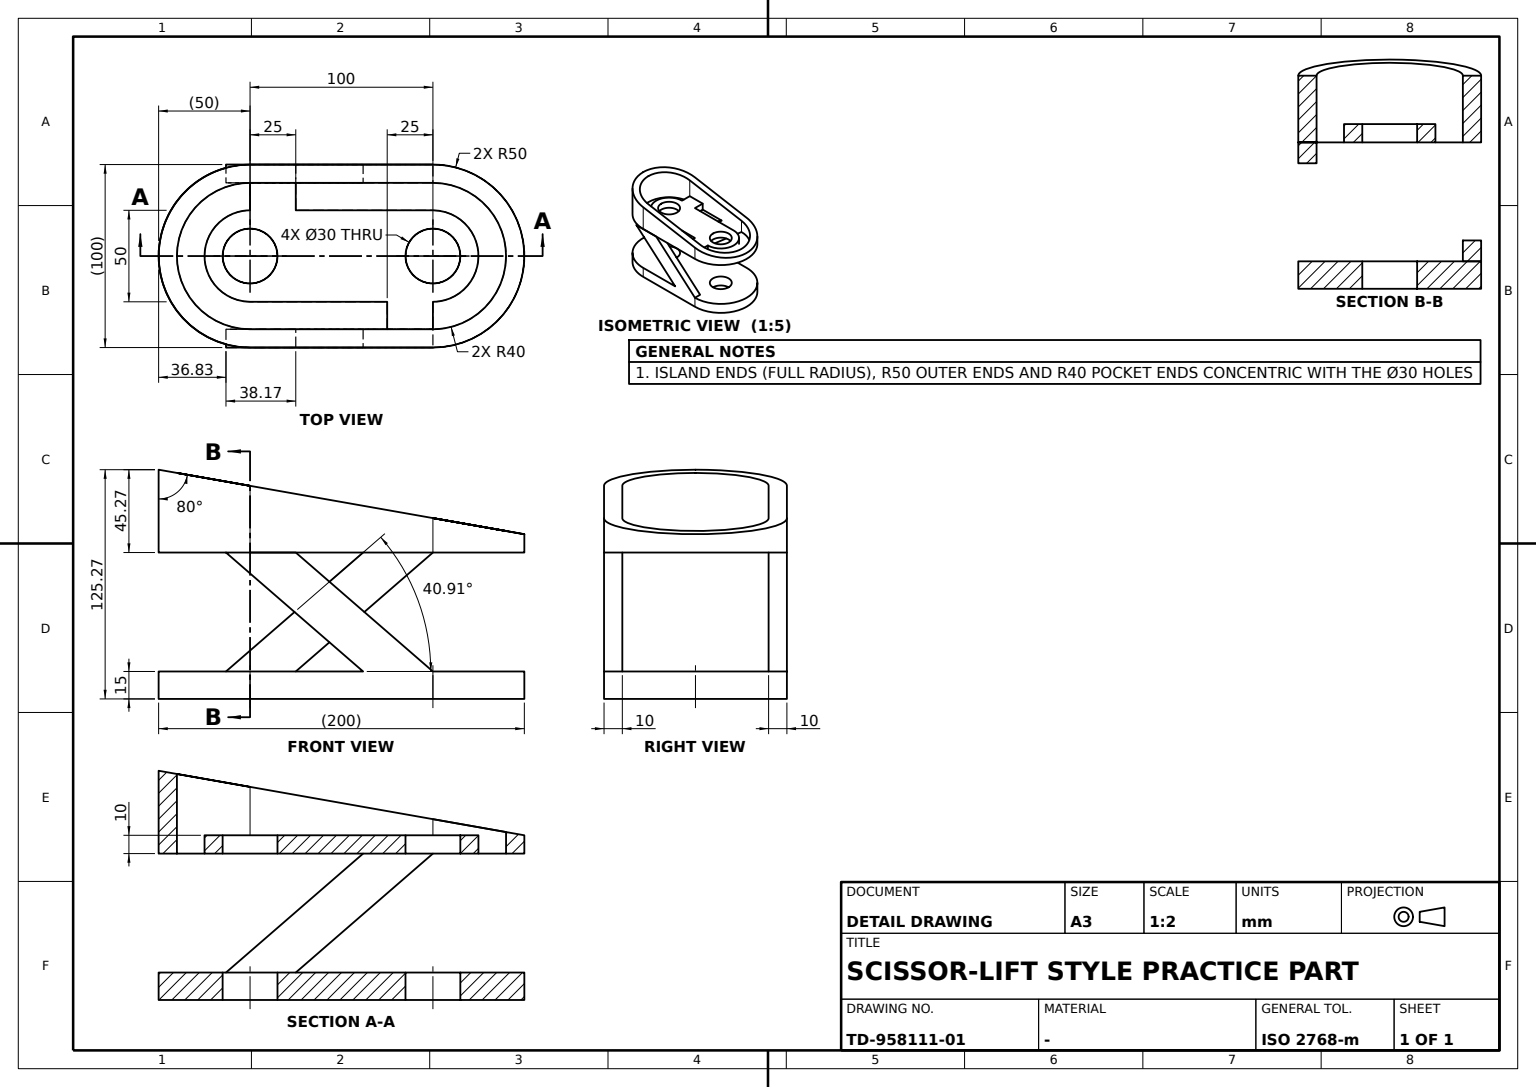
ISO-10303-21;
HEADER;
FILE_DESCRIPTION((''),'2;1');
FILE_NAME('','',(''),(''),'','','');
FILE_SCHEMA(('AUTOMOTIVE_DESIGN'));
ENDSEC;
DATA;
#1=APPLICATION_CONTEXT('');
#2=PRODUCT_CONTEXT('',#1,'mechanical');
#3=PRODUCT('','','',(#2));
#4=PRODUCT_DEFINITION_FORMATION('','',#3);
#5=PRODUCT_DEFINITION_CONTEXT('',#1,'design');
#6=PRODUCT_DEFINITION('','',#4,#5);
#7=PRODUCT_DEFINITION_SHAPE('','',#6);
#8=(LENGTH_UNIT()NAMED_UNIT(*)SI_UNIT(.MILLI.,.METRE.));
#9=(NAMED_UNIT(*)PLANE_ANGLE_UNIT()SI_UNIT($,.RADIAN.));
#10=(NAMED_UNIT(*)SI_UNIT($,.STERADIAN.)SOLID_ANGLE_UNIT());
#11=UNCERTAINTY_MEASURE_WITH_UNIT(LENGTH_MEASURE(0.005),#8,'distance_accuracy_value','');
#12=(GEOMETRIC_REPRESENTATION_CONTEXT(3)GLOBAL_UNCERTAINTY_ASSIGNED_CONTEXT((#11))GLOBAL_UNIT_ASSIGNED_CONTEXT((#8,#9,#10))REPRESENTATION_CONTEXT('',''));
#13=CARTESIAN_POINT('',(50.,-50.,0.));
#14=VERTEX_POINT('',#13);
#15=CARTESIAN_POINT('',(100.,0.,0.));
#16=VERTEX_POINT('',#15);
#17=CARTESIAN_POINT('',(50.,0.,0.));
#18=DIRECTION('',(0.,0.,1.));
#19=DIRECTION('',(1.,0.,0.));
#20=AXIS2_PLACEMENT_3D('',#17,#18,#19);
#21=CIRCLE('',#20,50.);
#22=EDGE_CURVE('',#14,#16,#21,.T.);
#23=ORIENTED_EDGE('',*,*,#22,.F.);
#24=CARTESIAN_POINT('',(50.,-50.,-15.));
#25=VERTEX_POINT('',#24);
#26=VECTOR('',#18,1000.);
#27=LINE('',#24,#26);
#28=EDGE_CURVE('',#25,#14,#27,.T.);
#29=ORIENTED_EDGE('',*,*,#28,.F.);
#30=CARTESIAN_POINT('',(100.,0.,-15.));
#31=VERTEX_POINT('',#30);
#32=CARTESIAN_POINT('',(50.,0.,-15.));
#33=AXIS2_PLACEMENT_3D('',#32,#18,#19);
#34=CIRCLE('',#33,50.);
#35=EDGE_CURVE('',#25,#31,#34,.T.);
#36=ORIENTED_EDGE('',*,*,#35,.T.);
#37=LINE('',#30,#26);
#38=EDGE_CURVE('',#31,#16,#37,.T.);
#39=ORIENTED_EDGE('',*,*,#38,.T.);
#40=EDGE_LOOP('',(#23,#29,#36,#39));
#41=FACE_BOUND('',#40,.T.);
#42=CYLINDRICAL_SURFACE('',#33,50.);
#43=ADVANCED_FACE('',(#41),#42,.T.);
#44=CARTESIAN_POINT('',(-65.,0.,0.));
#45=VERTEX_POINT('',#44);
#46=CARTESIAN_POINT('',(-35.,0.,0.));
#47=VERTEX_POINT('',#46);
#48=CARTESIAN_POINT('',(-50.,0.,0.));
#49=AXIS2_PLACEMENT_3D('',#48,#18,#19);
#50=CIRCLE('',#49,15.);
#51=EDGE_CURVE('',#45,#47,#50,.T.);
#52=ORIENTED_EDGE('',*,*,#51,.T.);
#53=CARTESIAN_POINT('',(-35.,0.,-15.));
#54=VERTEX_POINT('',#53);
#55=LINE('',#53,#26);
#56=EDGE_CURVE('',#54,#47,#55,.T.);
#57=ORIENTED_EDGE('',*,*,#56,.F.);
#58=CARTESIAN_POINT('',(-65.,0.,-15.));
#59=VERTEX_POINT('',#58);
#60=CARTESIAN_POINT('',(-50.,0.,-15.));
#61=AXIS2_PLACEMENT_3D('',#60,#18,#19);
#62=CIRCLE('',#61,15.);
#63=EDGE_CURVE('',#59,#54,#62,.T.);
#64=ORIENTED_EDGE('',*,*,#63,.F.);
#65=LINE('',#58,#26);
#66=EDGE_CURVE('',#45,#59,#65,.F.);
#67=ORIENTED_EDGE('',*,*,#66,.F.);
#68=EDGE_LOOP('',(#52,#57,#64,#67));
#69=FACE_BOUND('',#68,.T.);
#70=CYLINDRICAL_SURFACE('',#61,15.);
#71=ADVANCED_FACE('',(#69),#70,.F.);
#72=CARTESIAN_POINT('',(-63.171987,-50.,65.));
#73=VERTEX_POINT('',#72);
#74=CARTESIAN_POINT('',(11.828013,-50.,0.));
#75=VERTEX_POINT('',#74);
#76=DIRECTION('',(0.755689083,0.,-0.654930538));
#77=VECTOR('',#76,1000.);
#78=LINE('',#72,#77);
#79=EDGE_CURVE('',#73,#75,#78,.T.);
#80=ORIENTED_EDGE('',*,*,#79,.F.);
#81=CARTESIAN_POINT('',(-63.171987,-40.,65.));
#82=VERTEX_POINT('',#81);
#83=DIRECTION('',(0.,-1.,0.));
#84=VECTOR('',#83,1000.);
#85=LINE('',#81,#84);
#86=EDGE_CURVE('',#82,#73,#85,.T.);
#87=ORIENTED_EDGE('',*,*,#86,.F.);
#88=CARTESIAN_POINT('',(11.828013,-40.,0.));
#89=VERTEX_POINT('',#88);
#90=LINE('',#81,#77);
#91=EDGE_CURVE('',#82,#89,#90,.T.);
#92=ORIENTED_EDGE('',*,*,#91,.T.);
#93=LINE('',#88,#84);
#94=EDGE_CURVE('',#89,#75,#93,.T.);
#95=ORIENTED_EDGE('',*,*,#94,.T.);
#96=EDGE_LOOP('',(#80,#87,#92,#95));
#97=FACE_BOUND('',#96,.T.);
#98=DIRECTION('',(-0.654930538,0.,-0.755689083));
#99=DIRECTION('',(-0.755689083,0.,0.654930538));
#100=AXIS2_PLACEMENT_3D('',#81,#98,#99);
#101=PLANE('',#100);
#102=ADVANCED_FACE('',(#97),#101,.T.);
#103=CARTESIAN_POINT('',(50.,50.,-15.));
#104=VERTEX_POINT('',#103);
#105=CARTESIAN_POINT('',(-50.,50.,-15.));
#106=VERTEX_POINT('',#105);
#107=DIRECTION('',(-1.,0.,0.));
#108=VECTOR('',#107,1000.);
#109=LINE('',#103,#108);
#110=EDGE_CURVE('',#104,#106,#109,.T.);
#111=ORIENTED_EDGE('',*,*,#110,.T.);
#112=CARTESIAN_POINT('',(-50.,50.,0.));
#113=VERTEX_POINT('',#112);
#114=LINE('',#105,#26);
#115=EDGE_CURVE('',#106,#113,#114,.T.);
#116=ORIENTED_EDGE('',*,*,#115,.T.);
#117=CARTESIAN_POINT('',(50.,50.,0.));
#118=VERTEX_POINT('',#117);
#119=LINE('',#117,#108);
#120=EDGE_CURVE('',#118,#113,#119,.T.);
#121=ORIENTED_EDGE('',*,*,#120,.F.);
#122=LINE('',#103,#26);
#123=EDGE_CURVE('',#104,#118,#122,.T.);
#124=ORIENTED_EDGE('',*,*,#123,.F.);
#125=EDGE_LOOP('',(#111,#116,#121,#124));
#126=FACE_BOUND('',#125,.T.);
#127=DIRECTION('',(0.,1.,0.));
#128=AXIS2_PLACEMENT_3D('',#103,#127,#18);
#129=PLANE('',#128);
#130=ADVANCED_FACE('',(#126),#129,.T.);
#131=CARTESIAN_POINT('',(-50.,-50.,-15.));
#132=VERTEX_POINT('',#131);
#133=CIRCLE('',#61,50.);
#134=EDGE_CURVE('',#106,#132,#133,.T.);
#135=ORIENTED_EDGE('',*,*,#134,.T.);
#136=CARTESIAN_POINT('',(-50.,-50.,0.));
#137=VERTEX_POINT('',#136);
#138=LINE('',#131,#26);
#139=EDGE_CURVE('',#132,#137,#138,.T.);
#140=ORIENTED_EDGE('',*,*,#139,.T.);
#141=CIRCLE('',#49,50.);
#142=EDGE_CURVE('',#113,#137,#141,.T.);
#143=ORIENTED_EDGE('',*,*,#142,.F.);
#144=ORIENTED_EDGE('',*,*,#115,.F.);
#145=EDGE_LOOP('',(#135,#140,#143,#144));
#146=FACE_BOUND('',#145,.T.);
#147=CYLINDRICAL_SURFACE('',#61,50.);
#148=ADVANCED_FACE('',(#146),#147,.T.);
#149=CARTESIAN_POINT('',(65.,0.,0.));
#150=VERTEX_POINT('',#149);
#151=CARTESIAN_POINT('',(35.,0.,0.));
#152=VERTEX_POINT('',#151);
#153=CIRCLE('',#20,15.);
#154=EDGE_CURVE('',#150,#152,#153,.T.);
#155=ORIENTED_EDGE('',*,*,#154,.T.);
#156=CARTESIAN_POINT('',(35.,0.,-15.));
#157=VERTEX_POINT('',#156);
#158=LINE('',#156,#26);
#159=EDGE_CURVE('',#152,#157,#158,.F.);
#160=ORIENTED_EDGE('',*,*,#159,.T.);
#161=CARTESIAN_POINT('',(65.,0.,-15.));
#162=VERTEX_POINT('',#161);
#163=CIRCLE('',#33,15.);
#164=EDGE_CURVE('',#162,#157,#163,.T.);
#165=ORIENTED_EDGE('',*,*,#164,.F.);
#166=LINE('',#161,#26);
#167=EDGE_CURVE('',#162,#150,#166,.T.);
#168=ORIENTED_EDGE('',*,*,#167,.T.);
#169=EDGE_LOOP('',(#155,#160,#165,#168));
#170=FACE_BOUND('',#169,.T.);
#171=CYLINDRICAL_SURFACE('',#33,15.);
#172=ADVANCED_FACE('',(#170),#171,.F.);
#173=CARTESIAN_POINT('',(-25.,-50.,65.));
#174=VERTEX_POINT('',#173);
#175=LINE('',#173,#108);
#176=EDGE_CURVE('',#174,#73,#175,.T.);
#177=ORIENTED_EDGE('',*,*,#176,.F.);
#178=CARTESIAN_POINT('',(-25.,-40.,65.));
#179=VERTEX_POINT('',#178);
#180=LINE('',#178,#84);
#181=EDGE_CURVE('',#179,#174,#180,.T.);
#182=ORIENTED_EDGE('',*,*,#181,.F.);
#183=LINE('',#178,#108);
#184=EDGE_CURVE('',#179,#82,#183,.T.);
#185=ORIENTED_EDGE('',*,*,#184,.T.);
#186=ORIENTED_EDGE('',*,*,#86,.T.);
#187=EDGE_LOOP('',(#177,#182,#185,#186));
#188=FACE_BOUND('',#187,.T.);
#189=AXIS2_PLACEMENT_3D('',#178,#18,#19);
#190=PLANE('',#189);
#191=ADVANCED_FACE('',(#188),#190,.T.);
#192=ORIENTED_EDGE('',*,*,#181,.T.);
#193=VECTOR('',#99,1000.);
#194=LINE('',#13,#193);
#195=EDGE_CURVE('',#14,#174,#194,.T.);
#196=ORIENTED_EDGE('',*,*,#195,.F.);
#197=CARTESIAN_POINT('',(50.,-40.,0.));
#198=VERTEX_POINT('',#197);
#199=LINE('',#197,#84);
#200=EDGE_CURVE('',#198,#14,#199,.T.);
#201=ORIENTED_EDGE('',*,*,#200,.F.);
#202=LINE('',#197,#193);
#203=EDGE_CURVE('',#198,#179,#202,.T.);
#204=ORIENTED_EDGE('',*,*,#203,.T.);
#205=EDGE_LOOP('',(#192,#196,#201,#204));
#206=FACE_BOUND('',#205,.T.);
#207=DIRECTION('',(0.654930538,0.,0.755689083));
#208=AXIS2_PLACEMENT_3D('',#197,#207,#76);
#209=PLANE('',#208);
#210=ADVANCED_FACE('',(#206),#209,.T.);
#211=EDGE_CURVE('',#54,#59,#62,.T.);
#212=ORIENTED_EDGE('',*,*,#211,.T.);
#213=ORIENTED_EDGE('',*,*,#63,.T.);
#214=EDGE_LOOP('',(#212,#213));
#215=FACE_BOUND('',#214,.T.);
#216=ORIENTED_EDGE('',*,*,#35,.F.);
#217=VECTOR('',#19,1000.);
#218=LINE('',#131,#217);
#219=EDGE_CURVE('',#132,#25,#218,.T.);
#220=ORIENTED_EDGE('',*,*,#219,.F.);
#221=ORIENTED_EDGE('',*,*,#134,.F.);
#222=ORIENTED_EDGE('',*,*,#110,.F.);
#223=EDGE_CURVE('',#31,#104,#34,.T.);
#224=ORIENTED_EDGE('',*,*,#223,.F.);
#225=EDGE_LOOP('',(#216,#220,#221,#222,#224));
#226=FACE_BOUND('',#225,.T.);
#227=EDGE_CURVE('',#157,#162,#163,.T.);
#228=ORIENTED_EDGE('',*,*,#227,.T.);
#229=ORIENTED_EDGE('',*,*,#164,.T.);
#230=EDGE_LOOP('',(#228,#229));
#231=FACE_BOUND('',#230,.T.);
#232=PLANE('',#61);
#233=ADVANCED_FACE('',(#215,#226,#231),#232,.F.);
#234=ORIENTED_EDGE('',*,*,#120,.T.);
#235=ORIENTED_EDGE('',*,*,#142,.T.);
#236=LINE('',#136,#217);
#237=EDGE_CURVE('',#137,#75,#236,.T.);
#238=ORIENTED_EDGE('',*,*,#237,.T.);
#239=ORIENTED_EDGE('',*,*,#94,.F.);
#240=LINE('',#88,#217);
#241=EDGE_CURVE('',#89,#198,#240,.T.);
#242=ORIENTED_EDGE('',*,*,#241,.T.);
#243=ORIENTED_EDGE('',*,*,#200,.T.);
#244=ORIENTED_EDGE('',*,*,#22,.T.);
#245=EDGE_CURVE('',#16,#118,#21,.T.);
#246=ORIENTED_EDGE('',*,*,#245,.T.);
#247=EDGE_LOOP('',(#234,#235,#238,#239,#242,#243,#244,#246));
#248=FACE_BOUND('',#247,.T.);
#249=ORIENTED_EDGE('',*,*,#51,.F.);
#250=EDGE_CURVE('',#47,#45,#50,.T.);
#251=ORIENTED_EDGE('',*,*,#250,.F.);
#252=EDGE_LOOP('',(#249,#251));
#253=FACE_BOUND('',#252,.T.);
#254=ORIENTED_EDGE('',*,*,#154,.F.);
#255=EDGE_CURVE('',#152,#150,#153,.T.);
#256=ORIENTED_EDGE('',*,*,#255,.F.);
#257=EDGE_LOOP('',(#254,#256));
#258=FACE_BOUND('',#257,.T.);
#259=PLANE('',#49);
#260=ADVANCED_FACE('',(#248,#253,#258),#259,.T.);
#261=ORIENTED_EDGE('',*,*,#123,.T.);
#262=ORIENTED_EDGE('',*,*,#245,.F.);
#263=ORIENTED_EDGE('',*,*,#38,.F.);
#264=ORIENTED_EDGE('',*,*,#223,.T.);
#265=EDGE_LOOP('',(#261,#262,#263,#264));
#266=FACE_BOUND('',#265,.T.);
#267=ADVANCED_FACE('',(#266),#42,.T.);
#268=ORIENTED_EDGE('',*,*,#167,.F.);
#269=ORIENTED_EDGE('',*,*,#227,.F.);
#270=ORIENTED_EDGE('',*,*,#159,.F.);
#271=ORIENTED_EDGE('',*,*,#255,.T.);
#272=EDGE_LOOP('',(#268,#269,#270,#271));
#273=FACE_BOUND('',#272,.T.);
#274=ADVANCED_FACE('',(#273),#171,.F.);
#275=ORIENTED_EDGE('',*,*,#56,.T.);
#276=ORIENTED_EDGE('',*,*,#250,.T.);
#277=ORIENTED_EDGE('',*,*,#66,.T.);
#278=ORIENTED_EDGE('',*,*,#211,.F.);
#279=EDGE_LOOP('',(#275,#276,#277,#278));
#280=FACE_BOUND('',#279,.T.);
#281=ADVANCED_FACE('',(#280),#70,.F.);
#282=ORIENTED_EDGE('',*,*,#28,.T.);
#283=ORIENTED_EDGE('',*,*,#195,.T.);
#284=ORIENTED_EDGE('',*,*,#176,.T.);
#285=ORIENTED_EDGE('',*,*,#79,.T.);
#286=ORIENTED_EDGE('',*,*,#237,.F.);
#287=ORIENTED_EDGE('',*,*,#139,.F.);
#288=ORIENTED_EDGE('',*,*,#219,.T.);
#289=EDGE_LOOP('',(#282,#283,#284,#285,#286,#287,#288));
#290=FACE_BOUND('',#289,.T.);
#291=DIRECTION('',(0.,0.,-1.));
#292=AXIS2_PLACEMENT_3D('',#131,#83,#291);
#293=PLANE('',#292);
#294=ADVANCED_FACE('',(#290),#293,.T.);
#295=ORIENTED_EDGE('',*,*,#241,.F.);
#296=ORIENTED_EDGE('',*,*,#91,.F.);
#297=ORIENTED_EDGE('',*,*,#184,.F.);
#298=ORIENTED_EDGE('',*,*,#203,.F.);
#299=EDGE_LOOP('',(#295,#296,#297,#298));
#300=FACE_BOUND('',#299,.T.);
#301=CARTESIAN_POINT('',(0.,-40.,0.));
#302=AXIS2_PLACEMENT_3D('',#301,#83,#291);
#303=PLANE('',#302);
#304=ADVANCED_FACE('',(#300),#303,.F.);
#305=CLOSED_SHELL('',(#43,#71,#102,#130,#148,#172,#191,#210,#233,#260,#267,#274,#281,#294,#304));
#306=MANIFOLD_SOLID_BREP('',#305);
#307=CARTESIAN_POINT('',(35.,0.,75.));
#308=VERTEX_POINT('',#307);
#309=CARTESIAN_POINT('',(65.,0.,75.));
#310=VERTEX_POINT('',#309);
#311=CARTESIAN_POINT('',(50.,0.,75.));
#312=AXIS2_PLACEMENT_3D('',#311,#18,#19);
#313=CIRCLE('',#312,15.);
#314=EDGE_CURVE('',#308,#310,#313,.T.);
#315=ORIENTED_EDGE('',*,*,#314,.T.);
#316=CARTESIAN_POINT('',(65.,0.,65.));
#317=VERTEX_POINT('',#316);
#318=LINE('',#316,#26);
#319=EDGE_CURVE('',#310,#317,#318,.F.);
#320=ORIENTED_EDGE('',*,*,#319,.T.);
#321=CARTESIAN_POINT('',(35.,0.,65.));
#322=VERTEX_POINT('',#321);
#323=CARTESIAN_POINT('',(50.,0.,65.));
#324=AXIS2_PLACEMENT_3D('',#323,#18,#19);
#325=CIRCLE('',#324,15.);
#326=EDGE_CURVE('',#322,#317,#325,.T.);
#327=ORIENTED_EDGE('',*,*,#326,.F.);
#328=LINE('',#321,#26);
#329=EDGE_CURVE('',#322,#308,#328,.T.);
#330=ORIENTED_EDGE('',*,*,#329,.T.);
#331=EDGE_LOOP('',(#315,#320,#327,#330));
#332=FACE_BOUND('',#331,.T.);
#333=CYLINDRICAL_SURFACE('',#324,15.);
#334=ADVANCED_FACE('',(#332),#333,.F.);
#335=CARTESIAN_POINT('',(-63.171987,50.,0.));
#336=VERTEX_POINT('',#335);
#337=CARTESIAN_POINT('',(11.828013,50.,65.));
#338=VERTEX_POINT('',#337);
#339=DIRECTION('',(0.755689083,0.,0.654930538));
#340=VECTOR('',#339,1000.);
#341=LINE('',#335,#340);
#342=EDGE_CURVE('',#336,#338,#341,.T.);
#343=ORIENTED_EDGE('',*,*,#342,.F.);
#344=CARTESIAN_POINT('',(-63.171987,40.,0.));
#345=VERTEX_POINT('',#344);
#346=VECTOR('',#127,1000.);
#347=LINE('',#344,#346);
#348=EDGE_CURVE('',#345,#336,#347,.T.);
#349=ORIENTED_EDGE('',*,*,#348,.F.);
#350=CARTESIAN_POINT('',(11.828013,40.,65.));
#351=VERTEX_POINT('',#350);
#352=LINE('',#344,#340);
#353=EDGE_CURVE('',#345,#351,#352,.T.);
#354=ORIENTED_EDGE('',*,*,#353,.T.);
#355=LINE('',#350,#346);
#356=EDGE_CURVE('',#351,#338,#355,.T.);
#357=ORIENTED_EDGE('',*,*,#356,.T.);
#358=EDGE_LOOP('',(#343,#349,#354,#357));
#359=FACE_BOUND('',#358,.T.);
#360=DIRECTION('',(-0.654930538,0.,0.755689083));
#361=AXIS2_PLACEMENT_3D('',#344,#360,#339);
#362=PLANE('',#361);
#363=ADVANCED_FACE('',(#359),#362,.T.);
#364=CARTESIAN_POINT('',(50.,40.,65.));
#365=VERTEX_POINT('',#364);
#366=CARTESIAN_POINT('',(50.,40.,83.816349));
#367=VERTEX_POINT('',#366);
#368=CARTESIAN_POINT('',(50.,40.,165.));
#369=LINE('',#368,#26);
#370=EDGE_CURVE('',#365,#367,#369,.T.);
#371=ORIENTED_EDGE('',*,*,#370,.T.);
#372=CARTESIAN_POINT('',(-50.,40.,101.449047));
#373=VERTEX_POINT('',#372);
#374=CARTESIAN_POINT('',(100.,40.,75.));
#375=DIRECTION('',(0.984807753,0.,-0.173648178));
#376=VECTOR('',#375,1000.);
#377=LINE('',#374,#376);
#378=EDGE_CURVE('',#373,#367,#377,.T.);
#379=ORIENTED_EDGE('',*,*,#378,.F.);
#380=CARTESIAN_POINT('',(-50.,40.,75.));
#381=VERTEX_POINT('',#380);
#382=CARTESIAN_POINT('',(-50.,40.,165.));
#383=LINE('',#382,#26);
#384=EDGE_CURVE('',#381,#373,#383,.T.);
#385=ORIENTED_EDGE('',*,*,#384,.F.);
#386=CARTESIAN_POINT('',(-25.,40.,75.));
#387=VERTEX_POINT('',#386);
#388=LINE('',#380,#217);
#389=EDGE_CURVE('',#381,#387,#388,.T.);
#390=ORIENTED_EDGE('',*,*,#389,.T.);
#391=CARTESIAN_POINT('',(-25.,40.,65.));
#392=VERTEX_POINT('',#391);
#393=VECTOR('',#291,1000.);
#394=LINE('',#386,#393);
#395=EDGE_CURVE('',#387,#392,#394,.T.);
#396=ORIENTED_EDGE('',*,*,#395,.T.);
#397=CARTESIAN_POINT('',(-50.,40.,65.));
#398=LINE('',#397,#217);
#399=EDGE_CURVE('',#392,#351,#398,.T.);
#400=ORIENTED_EDGE('',*,*,#399,.T.);
#401=ORIENTED_EDGE('',*,*,#353,.F.);
#402=CARTESIAN_POINT('',(-25.,40.,0.));
#403=VERTEX_POINT('',#402);
#404=LINE('',#402,#108);
#405=EDGE_CURVE('',#403,#345,#404,.T.);
#406=ORIENTED_EDGE('',*,*,#405,.F.);
#407=DIRECTION('',(-0.755689083,0.,-0.654930538));
#408=VECTOR('',#407,1000.);
#409=LINE('',#364,#408);
#410=EDGE_CURVE('',#365,#403,#409,.T.);
#411=ORIENTED_EDGE('',*,*,#410,.F.);
#412=EDGE_LOOP('',(#371,#379,#385,#390,#396,#400,#401,#406,#411));
#413=FACE_BOUND('',#412,.T.);
#414=AXIS2_PLACEMENT_3D('',#382,#127,#107);
#415=PLANE('',#414);
#416=ADVANCED_FACE('',(#413),#415,.F.);
#417=ORIENTED_EDGE('',*,*,#326,.T.);
#418=EDGE_CURVE('',#317,#322,#325,.T.);
#419=ORIENTED_EDGE('',*,*,#418,.T.);
#420=EDGE_LOOP('',(#417,#419));
#421=FACE_BOUND('',#420,.T.);
#422=CARTESIAN_POINT('',(-50.,50.,65.));
#423=VERTEX_POINT('',#422);
#424=CARTESIAN_POINT('',(-100.,0.,65.));
#425=VERTEX_POINT('',#424);
#426=CARTESIAN_POINT('',(-50.,0.,65.));
#427=AXIS2_PLACEMENT_3D('',#426,#18,#107);
#428=CIRCLE('',#427,50.);
#429=EDGE_CURVE('',#423,#425,#428,.T.);
#430=ORIENTED_EDGE('',*,*,#429,.F.);
#431=CARTESIAN_POINT('',(-100.,50.,65.));
#432=LINE('',#431,#217);
#433=EDGE_CURVE('',#423,#338,#432,.T.);
#434=ORIENTED_EDGE('',*,*,#433,.T.);
#435=ORIENTED_EDGE('',*,*,#356,.F.);
#436=ORIENTED_EDGE('',*,*,#399,.F.);
#437=CARTESIAN_POINT('',(-25.,25.,65.));
#438=VERTEX_POINT('',#437);
#439=LINE('',#391,#84);
#440=EDGE_CURVE('',#392,#438,#439,.T.);
#441=ORIENTED_EDGE('',*,*,#440,.T.);
#442=CARTESIAN_POINT('',(49.999991,24.996154,65.));
#443=VERTEX_POINT('',#442);
#444=CARTESIAN_POINT('',(-1.5625,25.,65.));
#445=CARTESIAN_POINT('',(23.4375,25.,65.));
#446=CARTESIAN_POINT('',(48.4375,25.,65.));
#447=B_SPLINE_CURVE_WITH_KNOTS('',3,(#437,#444,#445,#446,#442),.UNSPECIFIED.,.F.,.F.,(4,1,4),(0.,0.9375,1.),.UNSPECIFIED.);
#448=EDGE_CURVE('',#438,#443,#447,.T.);
#449=ORIENTED_EDGE('',*,*,#448,.T.);
#450=CARTESIAN_POINT('',(50.,-25.,65.));
#451=VERTEX_POINT('',#450);
#452=CARTESIAN_POINT('',(52.205057,24.990727,65.));
#453=CARTESIAN_POINT('',(61.613675,23.898962,65.));
#454=CARTESIAN_POINT('',(71.64521,17.462121,65.));
#455=CARTESIAN_POINT('',(74.895083,6.615231,65.));
#456=CARTESIAN_POINT('',(74.895083,-8.820307,65.));
#457=CARTESIAN_POINT('',(70.496911,-20.515589,65.));
#458=CARTESIAN_POINT('',(58.820229,-24.962906,65.));
#459=(BOUNDED_CURVE()B_SPLINE_CURVE(4,(#442,#452,#453,#454,#455,#456,#457,#458,#450),.UNSPECIFIED.,.F.,.F.)B_SPLINE_CURVE_WITH_KNOTS((5,1,3,5),(0.,0.125,0.5,1.),.UNSPECIFIED.)CURVE()GEOMETRIC_REPRESENTATION_ITEM()RATIONAL_B_SPLINE_CURVE((0.585277204,0.585277204,0.57699372,0.560426752,0.585277204,0.585277204,0.552143268,0.585277204,0.585277204))REPRESENTATION_ITEM(''));
#460=EDGE_CURVE('',#443,#451,#459,.T.);
#461=ORIENTED_EDGE('',*,*,#460,.T.);
#462=CARTESIAN_POINT('',(50.,-40.,65.));
#463=VERTEX_POINT('',#462);
#464=LINE('',#450,#84);
#465=EDGE_CURVE('',#451,#463,#464,.T.);
#466=ORIENTED_EDGE('',*,*,#465,.T.);
#467=AXIS2_PLACEMENT_3D('',#323,#291,#107);
#468=CIRCLE('',#467,40.);
#469=EDGE_CURVE('',#365,#463,#468,.T.);
#470=ORIENTED_EDGE('',*,*,#469,.F.);
#471=CARTESIAN_POINT('',(50.,50.,65.));
#472=VERTEX_POINT('',#471);
#473=LINE('',#364,#346);
#474=EDGE_CURVE('',#365,#472,#473,.T.);
#475=ORIENTED_EDGE('',*,*,#474,.T.);
#476=CARTESIAN_POINT('',(50.,-50.,65.));
#477=VERTEX_POINT('',#476);
#478=AXIS2_PLACEMENT_3D('',#323,#18,#107);
#479=CIRCLE('',#478,50.);
#480=EDGE_CURVE('',#477,#472,#479,.T.);
#481=ORIENTED_EDGE('',*,*,#480,.F.);
#482=CARTESIAN_POINT('',(-50.,-50.,65.));
#483=VERTEX_POINT('',#482);
#484=CARTESIAN_POINT('',(-100.,-50.,65.));
#485=LINE('',#484,#217);
#486=EDGE_CURVE('',#483,#477,#485,.T.);
#487=ORIENTED_EDGE('',*,*,#486,.F.);
#488=EDGE_CURVE('',#425,#483,#428,.T.);
#489=ORIENTED_EDGE('',*,*,#488,.F.);
#490=EDGE_LOOP('',(#430,#434,#435,#436,#441,#449,#461,#466,#470,#475,#481,#487,#489));
#491=FACE_BOUND('',#490,.T.);
#492=CARTESIAN_POINT('',(-50.,-40.,65.));
#493=VERTEX_POINT('',#492);
#494=CARTESIAN_POINT('',(-90.,0.,65.));
#495=VERTEX_POINT('',#494);
#496=AXIS2_PLACEMENT_3D('',#426,#291,#19);
#497=CIRCLE('',#496,40.);
#498=EDGE_CURVE('',#493,#495,#497,.T.);
#499=ORIENTED_EDGE('',*,*,#498,.F.);
#500=CARTESIAN_POINT('',(25.,-40.,65.));
#501=VERTEX_POINT('',#500);
#502=LINE('',#462,#108);
#503=EDGE_CURVE('',#501,#493,#502,.T.);
#504=ORIENTED_EDGE('',*,*,#503,.F.);
#505=CARTESIAN_POINT('',(25.,-25.,65.));
#506=VERTEX_POINT('',#505);
#507=LINE('',#500,#346);
#508=EDGE_CURVE('',#501,#506,#507,.T.);
#509=ORIENTED_EDGE('',*,*,#508,.T.);
#510=CARTESIAN_POINT('',(-49.999991,-24.996154,65.));
#511=VERTEX_POINT('',#510);
#512=CARTESIAN_POINT('',(1.5625,-25.,65.));
#513=CARTESIAN_POINT('',(-23.4375,-25.,65.));
#514=CARTESIAN_POINT('',(-48.4375,-25.,65.));
#515=B_SPLINE_CURVE_WITH_KNOTS('',3,(#505,#512,#513,#514,#510),.UNSPECIFIED.,.F.,.F.,(4,1,4),(0.,0.9375,1.),.UNSPECIFIED.);
#516=EDGE_CURVE('',#506,#511,#515,.T.);
#517=ORIENTED_EDGE('',*,*,#516,.T.);
#518=CARTESIAN_POINT('',(-50.,25.,65.));
#519=VERTEX_POINT('',#518);
#520=CARTESIAN_POINT('',(-52.205057,-24.990727,65.));
#521=CARTESIAN_POINT('',(-61.613675,-23.898962,65.));
#522=CARTESIAN_POINT('',(-71.64521,-17.462121,65.));
#523=CARTESIAN_POINT('',(-74.895083,-6.615231,65.));
#524=CARTESIAN_POINT('',(-74.895083,8.820307,65.));
#525=CARTESIAN_POINT('',(-70.496911,20.515589,65.));
#526=CARTESIAN_POINT('',(-58.820229,24.962906,65.));
#527=(BOUNDED_CURVE()B_SPLINE_CURVE(4,(#510,#520,#521,#522,#523,#524,#525,#526,#518),.UNSPECIFIED.,.F.,.F.)B_SPLINE_CURVE_WITH_KNOTS((5,1,3,5),(0.,0.125,0.5,1.),.UNSPECIFIED.)CURVE()GEOMETRIC_REPRESENTATION_ITEM()RATIONAL_B_SPLINE_CURVE((0.585277204,0.585277204,0.57699372,0.560426752,0.585277204,0.585277204,0.552143268,0.585277204,0.585277204))REPRESENTATION_ITEM(''));
#528=EDGE_CURVE('',#511,#519,#527,.T.);
#529=ORIENTED_EDGE('',*,*,#528,.T.);
#530=VERTEX_POINT('',#397);
#531=LINE('',#518,#346);
#532=EDGE_CURVE('',#519,#530,#531,.T.);
#533=ORIENTED_EDGE('',*,*,#532,.T.);
#534=EDGE_CURVE('',#495,#530,#497,.T.);
#535=ORIENTED_EDGE('',*,*,#534,.F.);
#536=EDGE_LOOP('',(#499,#504,#509,#517,#529,#533,#535));
#537=FACE_BOUND('',#536,.T.);
#538=CARTESIAN_POINT('',(-65.,0.,65.));
#539=VERTEX_POINT('',#538);
#540=CARTESIAN_POINT('',(-35.,0.,65.));
#541=VERTEX_POINT('',#540);
#542=AXIS2_PLACEMENT_3D('',#426,#18,#19);
#543=CIRCLE('',#542,15.);
#544=EDGE_CURVE('',#539,#541,#543,.T.);
#545=ORIENTED_EDGE('',*,*,#544,.T.);
#546=EDGE_CURVE('',#541,#539,#543,.T.);
#547=ORIENTED_EDGE('',*,*,#546,.T.);
#548=EDGE_LOOP('',(#545,#547));
#549=FACE_BOUND('',#548,.T.);
#550=AXIS2_PLACEMENT_3D('',#484,#18,#19);
#551=PLANE('',#550);
#552=ADVANCED_FACE('',(#421,#491,#537,#549),#551,.F.);
#553=CARTESIAN_POINT('',(-100.,0.,110.265396));
#554=VERTEX_POINT('',#553);
#555=CARTESIAN_POINT('',(-100.,0.,165.));
#556=LINE('',#555,#393);
#557=EDGE_CURVE('',#554,#425,#556,.T.);
#558=ORIENTED_EDGE('',*,*,#557,.F.);
#559=CARTESIAN_POINT('',(-50.,50.,101.449047));
#560=VERTEX_POINT('',#559);
#561=CARTESIAN_POINT('',(-79.289322,50.,106.613545));
#562=CARTESIAN_POINT('',(-100.,29.289322,110.265396));
#563=(BOUNDED_CURVE()B_SPLINE_CURVE(3,(#559,#561,#562,#553),.UNSPECIFIED.,.F.,.F.)B_SPLINE_CURVE_WITH_KNOTS((4,4),(1.570796327,3.141592654),.UNSPECIFIED.)CURVE()GEOMETRIC_REPRESENTATION_ITEM()RATIONAL_B_SPLINE_CURVE((1.,0.804737854,0.804737854,1.))REPRESENTATION_ITEM(''));
#564=EDGE_CURVE('',#560,#554,#563,.T.);
#565=ORIENTED_EDGE('',*,*,#564,.F.);
#566=CARTESIAN_POINT('',(-50.,50.,165.));
#567=LINE('',#566,#393);
#568=EDGE_CURVE('',#560,#423,#567,.T.);
#569=ORIENTED_EDGE('',*,*,#568,.T.);
#570=ORIENTED_EDGE('',*,*,#429,.T.);
#571=EDGE_LOOP('',(#558,#565,#569,#570));
#572=FACE_BOUND('',#571,.T.);
#573=CARTESIAN_POINT('',(-50.,0.,165.));
#574=AXIS2_PLACEMENT_3D('',#573,#291,#107);
#575=CYLINDRICAL_SURFACE('',#574,50.);
#576=ADVANCED_FACE('',(#572),#575,.T.);
#577=ORIENTED_EDGE('',*,*,#348,.T.);
#578=CARTESIAN_POINT('',(-25.,50.,0.));
#579=VERTEX_POINT('',#578);
#580=LINE('',#578,#108);
#581=EDGE_CURVE('',#579,#336,#580,.T.);
#582=ORIENTED_EDGE('',*,*,#581,.F.);
#583=LINE('',#402,#346);
#584=EDGE_CURVE('',#403,#579,#583,.T.);
#585=ORIENTED_EDGE('',*,*,#584,.F.);
#586=ORIENTED_EDGE('',*,*,#405,.T.);
#587=EDGE_LOOP('',(#577,#582,#585,#586));
#588=FACE_BOUND('',#587,.T.);
#589=AXIS2_PLACEMENT_3D('',#402,#291,#107);
#590=PLANE('',#589);
#591=ADVANCED_FACE('',(#588),#590,.T.);
#592=CARTESIAN_POINT('',(50.,-25.,75.));
#593=VERTEX_POINT('',#592);
#594=LINE('',#592,#393);
#595=EDGE_CURVE('',#593,#451,#594,.T.);
#596=ORIENTED_EDGE('',*,*,#595,.F.);
#597=CARTESIAN_POINT('',(50.,-40.,75.));
#598=VERTEX_POINT('',#597);
#599=LINE('',#592,#84);
#600=EDGE_CURVE('',#593,#598,#599,.T.);
#601=ORIENTED_EDGE('',*,*,#600,.T.);
#602=CARTESIAN_POINT('',(50.,-40.,165.));
#603=LINE('',#602,#26);
#604=EDGE_CURVE('',#463,#598,#603,.T.);
#605=ORIENTED_EDGE('',*,*,#604,.F.);
#606=ORIENTED_EDGE('',*,*,#465,.F.);
#607=EDGE_LOOP('',(#596,#601,#605,#606));
#608=FACE_BOUND('',#607,.T.);
#609=AXIS2_PLACEMENT_3D('',#592,#19,#127);
#610=PLANE('',#609);
#611=ADVANCED_FACE('',(#608),#610,.T.);
#612=CARTESIAN_POINT('',(25.,-25.,75.));
#613=VERTEX_POINT('',#612);
#614=LINE('',#612,#393);
#615=EDGE_CURVE('',#613,#506,#614,.T.);
#616=ORIENTED_EDGE('',*,*,#615,.T.);
#617=ORIENTED_EDGE('',*,*,#508,.F.);
#618=CARTESIAN_POINT('',(25.,-40.,75.));
#619=VERTEX_POINT('',#618);
#620=LINE('',#618,#393);
#621=EDGE_CURVE('',#619,#501,#620,.T.);
#622=ORIENTED_EDGE('',*,*,#621,.F.);
#623=LINE('',#618,#346);
#624=EDGE_CURVE('',#619,#613,#623,.T.);
#625=ORIENTED_EDGE('',*,*,#624,.T.);
#626=EDGE_LOOP('',(#616,#617,#622,#625));
#627=FACE_BOUND('',#626,.T.);
#628=AXIS2_PLACEMENT_3D('',#618,#107,#83);
#629=PLANE('',#628);
#630=ADVANCED_FACE('',(#627),#629,.T.);
#631=ORIENTED_EDGE('',*,*,#418,.F.);
#632=ORIENTED_EDGE('',*,*,#319,.F.);
#633=EDGE_CURVE('',#310,#308,#313,.T.);
#634=ORIENTED_EDGE('',*,*,#633,.T.);
#635=ORIENTED_EDGE('',*,*,#329,.F.);
#636=EDGE_LOOP('',(#631,#632,#634,#635));
#637=FACE_BOUND('',#636,.T.);
#638=ADVANCED_FACE('',(#637),#333,.F.);
#639=CARTESIAN_POINT('',(-49.999991,-24.996154,75.));
#640=VERTEX_POINT('',#639);
#641=LINE('',#639,#393);
#642=EDGE_CURVE('',#640,#511,#641,.T.);
#643=ORIENTED_EDGE('',*,*,#642,.F.);
#644=CARTESIAN_POINT('',(-50.,25.,75.));
#645=VERTEX_POINT('',#644);
#646=CARTESIAN_POINT('',(-52.205057,-24.990727,75.));
#647=CARTESIAN_POINT('',(-61.613675,-23.898962,75.));
#648=CARTESIAN_POINT('',(-71.64521,-17.462121,75.));
#649=CARTESIAN_POINT('',(-74.895083,-6.615231,75.));
#650=CARTESIAN_POINT('',(-74.895083,8.820307,75.));
#651=CARTESIAN_POINT('',(-70.496911,20.515589,75.));
#652=CARTESIAN_POINT('',(-58.820229,24.962906,75.));
#653=(BOUNDED_CURVE()B_SPLINE_CURVE(4,(#639,#646,#647,#648,#649,#650,#651,#652,#644),.UNSPECIFIED.,.F.,.F.)B_SPLINE_CURVE_WITH_KNOTS((5,1,3,5),(0.,0.125,0.5,1.),.UNSPECIFIED.)CURVE()GEOMETRIC_REPRESENTATION_ITEM()RATIONAL_B_SPLINE_CURVE((0.585277204,0.585277204,0.57699372,0.560426752,0.585277204,0.585277204,0.552143268,0.585277204,0.585277204))REPRESENTATION_ITEM(''));
#654=EDGE_CURVE('',#640,#645,#653,.T.);
#655=ORIENTED_EDGE('',*,*,#654,.T.);
#656=LINE('',#644,#393);
#657=EDGE_CURVE('',#645,#519,#656,.T.);
#658=ORIENTED_EDGE('',*,*,#657,.T.);
#659=ORIENTED_EDGE('',*,*,#528,.F.);
#660=EDGE_LOOP('',(#643,#655,#658,#659));
#661=FACE_BOUND('',#660,.T.);
#662=(BOUNDED_SURFACE()B_SPLINE_SURFACE(4,1,((#639,#510),(#646,#520),(#647,#521),(#648,#522),(#649,#523),(#650,#524),(#651,#525),(#652,#526),(#644,#518)),.SURF_OF_LINEAR_EXTRUSION.,.F.,.F.,.F.)B_SPLINE_SURFACE_WITH_KNOTS((5,1,3,5),(2,2),(0.,0.125,0.5,1.),(0.,1.),.UNSPECIFIED.)GEOMETRIC_REPRESENTATION_ITEM()RATIONAL_B_SPLINE_SURFACE(((0.585277204,0.585277204),(0.585277204,0.585277204),(0.57699372,0.57699372),(0.560426752,0.560426752),(0.585277204,0.585277204),(0.585277204,0.585277204),(0.552143268,0.552143268),(0.585277204,0.585277204),(0.585277204,0.585277204)))REPRESENTATION_ITEM('')SURFACE());
#663=ADVANCED_FACE('',(#661),#662,.T.);
#664=CARTESIAN_POINT('',(1.5625,-25.,75.));
#665=CARTESIAN_POINT('',(-23.4375,-25.,75.));
#666=CARTESIAN_POINT('',(-48.4375,-25.,75.));
#667=B_SPLINE_CURVE_WITH_KNOTS('',3,(#612,#664,#665,#666,#639),.UNSPECIFIED.,.F.,.F.,(4,1,4),(0.,0.9375,1.),.UNSPECIFIED.);
#668=EDGE_CURVE('',#613,#640,#667,.T.);
#669=ORIENTED_EDGE('',*,*,#668,.T.);
#670=ORIENTED_EDGE('',*,*,#642,.T.);
#671=ORIENTED_EDGE('',*,*,#516,.F.);
#672=ORIENTED_EDGE('',*,*,#615,.F.);
#673=EDGE_LOOP('',(#669,#670,#671,#672));
#674=FACE_BOUND('',#673,.T.);
#675=B_SPLINE_SURFACE_WITH_KNOTS('',3,1,((#612,#505),(#664,#512),(#665,#513),(#666,#514),(#639,#510)),.SURF_OF_LINEAR_EXTRUSION.,.F.,.F.,.F.,(4,1,4),(2,2),(0.,0.9375,1.),(0.,1.),.UNSPECIFIED.);
#676=ADVANCED_FACE('',(#674),#675,.T.);
#677=CARTESIAN_POINT('',(50.,-40.,83.816349));
#678=VERTEX_POINT('',#677);
#679=CARTESIAN_POINT('',(130.,40.,69.710191));
#680=CARTESIAN_POINT('',(130.,-40.,69.710191));
#681=(BOUNDED_CURVE()B_SPLINE_CURVE(3,(#366,#679,#680,#677),.UNSPECIFIED.,.F.,.F.)B_SPLINE_CURVE_WITH_KNOTS((4,4),(4.71238898,7.853981634),.UNSPECIFIED.)CURVE()GEOMETRIC_REPRESENTATION_ITEM()RATIONAL_B_SPLINE_CURVE((1.,0.333333333,0.333333333,1.))REPRESENTATION_ITEM(''));
#682=EDGE_CURVE('',#367,#678,#681,.T.);
#683=ORIENTED_EDGE('',*,*,#682,.F.);
#684=ORIENTED_EDGE('',*,*,#370,.F.);
#685=ORIENTED_EDGE('',*,*,#469,.T.);
#686=ORIENTED_EDGE('',*,*,#604,.T.);
#687=EDGE_CURVE('',#598,#678,#603,.T.);
#688=ORIENTED_EDGE('',*,*,#687,.T.);
#689=EDGE_LOOP('',(#683,#684,#685,#686,#688));
#690=FACE_BOUND('',#689,.T.);
#691=CARTESIAN_POINT('',(50.,0.,165.));
#692=AXIS2_PLACEMENT_3D('',#691,#291,#107);
#693=CYLINDRICAL_SURFACE('',#692,40.);
#694=ADVANCED_FACE('',(#690),#693,.F.);
#695=ORIENTED_EDGE('',*,*,#384,.T.);
#696=CARTESIAN_POINT('',(-90.,0.,108.502126));
#697=VERTEX_POINT('',#696);
#698=CARTESIAN_POINT('',(-90.,23.431458,108.502126));
#699=CARTESIAN_POINT('',(-73.431458,40.,105.580645));
#700=(BOUNDED_CURVE()B_SPLINE_CURVE(3,(#696,#698,#699,#372),.UNSPECIFIED.,.F.,.F.)B_SPLINE_CURVE_WITH_KNOTS((4,4),(3.141592654,4.71238898),.UNSPECIFIED.)CURVE()GEOMETRIC_REPRESENTATION_ITEM()RATIONAL_B_SPLINE_CURVE((1.,0.804737854,0.804737854,1.))REPRESENTATION_ITEM(''));
#701=EDGE_CURVE('',#697,#373,#700,.T.);
#702=ORIENTED_EDGE('',*,*,#701,.F.);
#703=CARTESIAN_POINT('',(-90.,0.,165.));
#704=LINE('',#703,#393);
#705=EDGE_CURVE('',#697,#495,#704,.T.);
#706=ORIENTED_EDGE('',*,*,#705,.T.);
#707=ORIENTED_EDGE('',*,*,#534,.T.);
#708=EDGE_CURVE('',#530,#381,#383,.T.);
#709=ORIENTED_EDGE('',*,*,#708,.T.);
#710=EDGE_LOOP('',(#695,#702,#706,#707,#709));
#711=FACE_BOUND('',#710,.T.);
#712=CYLINDRICAL_SURFACE('',#574,40.);
#713=ADVANCED_FACE('',(#711),#712,.F.);
#714=ORIENTED_EDGE('',*,*,#474,.F.);
#715=ORIENTED_EDGE('',*,*,#410,.T.);
#716=ORIENTED_EDGE('',*,*,#584,.T.);
#717=LINE('',#471,#408);
#718=EDGE_CURVE('',#472,#579,#717,.T.);
#719=ORIENTED_EDGE('',*,*,#718,.F.);
#720=EDGE_LOOP('',(#714,#715,#716,#719));
#721=FACE_BOUND('',#720,.T.);
#722=DIRECTION('',(0.654930538,0.,-0.755689083));
#723=AXIS2_PLACEMENT_3D('',#364,#722,#407);
#724=PLANE('',#723);
#725=ADVANCED_FACE('',(#721),#724,.T.);
#726=CARTESIAN_POINT('',(-65.,0.,75.));
#727=VERTEX_POINT('',#726);
#728=LINE('',#538,#26);
#729=EDGE_CURVE('',#539,#727,#728,.T.);
#730=ORIENTED_EDGE('',*,*,#729,.T.);
#731=CARTESIAN_POINT('',(-35.,0.,75.));
#732=VERTEX_POINT('',#731);
#733=CARTESIAN_POINT('',(-50.,0.,75.));
#734=AXIS2_PLACEMENT_3D('',#733,#18,#19);
#735=CIRCLE('',#734,15.);
#736=EDGE_CURVE('',#727,#732,#735,.T.);
#737=ORIENTED_EDGE('',*,*,#736,.T.);
#738=LINE('',#540,#26);
#739=EDGE_CURVE('',#732,#541,#738,.F.);
#740=ORIENTED_EDGE('',*,*,#739,.T.);
#741=ORIENTED_EDGE('',*,*,#544,.F.);
#742=EDGE_LOOP('',(#730,#737,#740,#741));
#743=FACE_BOUND('',#742,.T.);
#744=CYLINDRICAL_SURFACE('',#542,15.);
#745=ADVANCED_FACE('',(#743),#744,.F.);
#746=CARTESIAN_POINT('',(-50.,-50.,101.449047));
#747=VERTEX_POINT('',#746);
#748=CARTESIAN_POINT('',(-50.,-50.,165.));
#749=LINE('',#748,#393);
#750=EDGE_CURVE('',#747,#483,#749,.T.);
#751=ORIENTED_EDGE('',*,*,#750,.F.);
#752=CARTESIAN_POINT('',(-100.,-29.289322,110.265396));
#753=CARTESIAN_POINT('',(-79.289322,-50.,106.613545));
#754=(BOUNDED_CURVE()B_SPLINE_CURVE(3,(#553,#752,#753,#746),.UNSPECIFIED.,.F.,.F.)B_SPLINE_CURVE_WITH_KNOTS((4,4),(3.141592654,4.71238898),.UNSPECIFIED.)CURVE()GEOMETRIC_REPRESENTATION_ITEM()RATIONAL_B_SPLINE_CURVE((1.,0.804737854,0.804737854,1.))REPRESENTATION_ITEM(''));
#755=EDGE_CURVE('',#554,#747,#754,.T.);
#756=ORIENTED_EDGE('',*,*,#755,.F.);
#757=ORIENTED_EDGE('',*,*,#557,.T.);
#758=ORIENTED_EDGE('',*,*,#488,.T.);
#759=EDGE_LOOP('',(#751,#756,#757,#758));
#760=FACE_BOUND('',#759,.T.);
#761=ADVANCED_FACE('',(#760),#575,.T.);
#762=CARTESIAN_POINT('',(-25.,25.,75.));
#763=VERTEX_POINT('',#762);
#764=LINE('',#762,#393);
#765=EDGE_CURVE('',#763,#438,#764,.T.);
#766=ORIENTED_EDGE('',*,*,#765,.T.);
#767=ORIENTED_EDGE('',*,*,#440,.F.);
#768=ORIENTED_EDGE('',*,*,#395,.F.);
#769=LINE('',#386,#84);
#770=EDGE_CURVE('',#387,#763,#769,.T.);
#771=ORIENTED_EDGE('',*,*,#770,.T.);
#772=EDGE_LOOP('',(#766,#767,#768,#771));
#773=FACE_BOUND('',#772,.T.);
#774=AXIS2_PLACEMENT_3D('',#386,#19,#127);
#775=PLANE('',#774);
#776=ADVANCED_FACE('',(#773),#775,.T.);
#777=CARTESIAN_POINT('',(-50.,-40.,101.449047));
#778=VERTEX_POINT('',#777);
#779=CARTESIAN_POINT('',(-73.431458,-40.,105.580645));
#780=CARTESIAN_POINT('',(-90.,-23.431458,108.502126));
#781=(BOUNDED_CURVE()B_SPLINE_CURVE(3,(#777,#779,#780,#696),.UNSPECIFIED.,.F.,.F.)B_SPLINE_CURVE_WITH_KNOTS((4,4),(1.570796327,3.141592654),.UNSPECIFIED.)CURVE()GEOMETRIC_REPRESENTATION_ITEM()RATIONAL_B_SPLINE_CURVE((1.,0.804737854,0.804737854,1.))REPRESENTATION_ITEM(''));
#782=EDGE_CURVE('',#778,#697,#781,.T.);
#783=ORIENTED_EDGE('',*,*,#782,.T.);
#784=ORIENTED_EDGE('',*,*,#701,.T.);
#785=ORIENTED_EDGE('',*,*,#378,.T.);
#786=ORIENTED_EDGE('',*,*,#682,.T.);
#787=CARTESIAN_POINT('',(100.,-40.,75.));
#788=DIRECTION('',(-0.984807753,0.,0.173648178));
#789=VECTOR('',#788,1000.);
#790=LINE('',#787,#789);
#791=EDGE_CURVE('',#678,#778,#790,.T.);
#792=ORIENTED_EDGE('',*,*,#791,.T.);
#793=EDGE_LOOP('',(#783,#784,#785,#786,#792));
#794=FACE_BOUND('',#793,.T.);
#795=CARTESIAN_POINT('',(50.,-50.,83.816349));
#796=VERTEX_POINT('',#795);
#797=CARTESIAN_POINT('',(50.,50.,83.816349));
#798=VERTEX_POINT('',#797);
#799=CARTESIAN_POINT('',(150.,-50.,66.183651));
#800=CARTESIAN_POINT('',(150.,50.,66.183651));
#801=(BOUNDED_CURVE()B_SPLINE_CURVE(3,(#795,#799,#800,#797),.UNSPECIFIED.,.F.,.F.)B_SPLINE_CURVE_WITH_KNOTS((4,4),(4.71238898,7.853981634),.UNSPECIFIED.)CURVE()GEOMETRIC_REPRESENTATION_ITEM()RATIONAL_B_SPLINE_CURVE((1.,0.333333333,0.333333333,1.))REPRESENTATION_ITEM(''));
#802=EDGE_CURVE('',#796,#798,#801,.T.);
#803=ORIENTED_EDGE('',*,*,#802,.T.);
#804=CARTESIAN_POINT('',(100.,50.,75.));
#805=LINE('',#804,#789);
#806=EDGE_CURVE('',#798,#560,#805,.T.);
#807=ORIENTED_EDGE('',*,*,#806,.T.);
#808=ORIENTED_EDGE('',*,*,#564,.T.);
#809=ORIENTED_EDGE('',*,*,#755,.T.);
#810=CARTESIAN_POINT('',(100.,-50.,75.));
#811=LINE('',#810,#789);
#812=EDGE_CURVE('',#796,#747,#811,.T.);
#813=ORIENTED_EDGE('',*,*,#812,.F.);
#814=EDGE_LOOP('',(#803,#807,#808,#809,#813));
#815=FACE_BOUND('',#814,.T.);
#816=DIRECTION('',(-0.173648178,0.,-0.984807753));
#817=AXIS2_PLACEMENT_3D('',#810,#816,#788);
#818=PLANE('',#817);
#819=ADVANCED_FACE('',(#794,#815),#818,.F.);
#820=EDGE_CURVE('',#732,#727,#735,.T.);
#821=ORIENTED_EDGE('',*,*,#820,.F.);
#822=ORIENTED_EDGE('',*,*,#736,.F.);
#823=EDGE_LOOP('',(#821,#822));
#824=FACE_BOUND('',#823,.T.);
#825=LINE('',#644,#346);
#826=EDGE_CURVE('',#645,#381,#825,.T.);
#827=ORIENTED_EDGE('',*,*,#826,.F.);
#828=ORIENTED_EDGE('',*,*,#654,.F.);
#829=ORIENTED_EDGE('',*,*,#668,.F.);
#830=ORIENTED_EDGE('',*,*,#624,.F.);
#831=LINE('',#597,#108);
#832=EDGE_CURVE('',#598,#619,#831,.T.);
#833=ORIENTED_EDGE('',*,*,#832,.F.);
#834=ORIENTED_EDGE('',*,*,#600,.F.);
#835=CARTESIAN_POINT('',(49.999991,24.996154,75.));
#836=VERTEX_POINT('',#835);
#837=CARTESIAN_POINT('',(52.205057,24.990727,75.));
#838=CARTESIAN_POINT('',(61.613675,23.898962,75.));
#839=CARTESIAN_POINT('',(71.64521,17.462121,75.));
#840=CARTESIAN_POINT('',(74.895083,6.615231,75.));
#841=CARTESIAN_POINT('',(74.895083,-8.820307,75.));
#842=CARTESIAN_POINT('',(70.496911,-20.515589,75.));
#843=CARTESIAN_POINT('',(58.820229,-24.962906,75.));
#844=(BOUNDED_CURVE()B_SPLINE_CURVE(4,(#835,#837,#838,#839,#840,#841,#842,#843,#592),.UNSPECIFIED.,.F.,.F.)B_SPLINE_CURVE_WITH_KNOTS((5,1,3,5),(0.,0.125,0.5,1.),.UNSPECIFIED.)CURVE()GEOMETRIC_REPRESENTATION_ITEM()RATIONAL_B_SPLINE_CURVE((0.585277204,0.585277204,0.57699372,0.560426752,0.585277204,0.585277204,0.552143268,0.585277204,0.585277204))REPRESENTATION_ITEM(''));
#845=EDGE_CURVE('',#836,#593,#844,.T.);
#846=ORIENTED_EDGE('',*,*,#845,.F.);
#847=CARTESIAN_POINT('',(-1.5625,25.,75.));
#848=CARTESIAN_POINT('',(23.4375,25.,75.));
#849=CARTESIAN_POINT('',(48.4375,25.,75.));
#850=B_SPLINE_CURVE_WITH_KNOTS('',3,(#762,#847,#848,#849,#835),.UNSPECIFIED.,.F.,.F.,(4,1,4),(0.,0.9375,1.),.UNSPECIFIED.);
#851=EDGE_CURVE('',#763,#836,#850,.T.);
#852=ORIENTED_EDGE('',*,*,#851,.F.);
#853=ORIENTED_EDGE('',*,*,#770,.F.);
#854=ORIENTED_EDGE('',*,*,#389,.F.);
#855=EDGE_LOOP('',(#827,#828,#829,#830,#833,#834,#846,#852,#853,#854));
#856=FACE_BOUND('',#855,.T.);
#857=ORIENTED_EDGE('',*,*,#314,.F.);
#858=ORIENTED_EDGE('',*,*,#633,.F.);
#859=EDGE_LOOP('',(#857,#858));
#860=FACE_BOUND('',#859,.T.);
#861=CARTESIAN_POINT('',(-74.895083,0.,75.));
#862=AXIS2_PLACEMENT_3D('',#861,#18,#19);
#863=PLANE('',#862);
#864=ADVANCED_FACE('',(#824,#856,#860),#863,.T.);
#865=ORIENTED_EDGE('',*,*,#532,.F.);
#866=ORIENTED_EDGE('',*,*,#657,.F.);
#867=ORIENTED_EDGE('',*,*,#826,.T.);
#868=ORIENTED_EDGE('',*,*,#708,.F.);
#869=EDGE_LOOP('',(#865,#866,#867,#868));
#870=FACE_BOUND('',#869,.T.);
#871=AXIS2_PLACEMENT_3D('',#644,#107,#83);
#872=PLANE('',#871);
#873=ADVANCED_FACE('',(#870),#872,.T.);
#874=CARTESIAN_POINT('',(-50.,-40.,165.));
#875=LINE('',#874,#26);
#876=EDGE_CURVE('',#493,#778,#875,.T.);
#877=ORIENTED_EDGE('',*,*,#876,.F.);
#878=ORIENTED_EDGE('',*,*,#498,.T.);
#879=ORIENTED_EDGE('',*,*,#705,.F.);
#880=ORIENTED_EDGE('',*,*,#782,.F.);
#881=EDGE_LOOP('',(#877,#878,#879,#880));
#882=FACE_BOUND('',#881,.T.);
#883=ADVANCED_FACE('',(#882),#712,.F.);
#884=ORIENTED_EDGE('',*,*,#460,.F.);
#885=LINE('',#835,#393);
#886=EDGE_CURVE('',#836,#443,#885,.T.);
#887=ORIENTED_EDGE('',*,*,#886,.F.);
#888=ORIENTED_EDGE('',*,*,#845,.T.);
#889=ORIENTED_EDGE('',*,*,#595,.T.);
#890=EDGE_LOOP('',(#884,#887,#888,#889));
#891=FACE_BOUND('',#890,.T.);
#892=(BOUNDED_SURFACE()B_SPLINE_SURFACE(4,1,((#835,#442),(#837,#452),(#838,#453),(#839,#454),(#840,#455),(#841,#456),(#842,#457),(#843,#458),(#592,#450)),.SURF_OF_LINEAR_EXTRUSION.,.F.,.F.,.F.)B_SPLINE_SURFACE_WITH_KNOTS((5,1,3,5),(2,2),(0.,0.125,0.5,1.),(0.,1.),.UNSPECIFIED.)GEOMETRIC_REPRESENTATION_ITEM()RATIONAL_B_SPLINE_SURFACE(((0.585277204,0.585277204),(0.585277204,0.585277204),(0.57699372,0.57699372),(0.560426752,0.560426752),(0.585277204,0.585277204),(0.585277204,0.585277204),(0.552143268,0.552143268),(0.585277204,0.585277204),(0.585277204,0.585277204)))REPRESENTATION_ITEM('')SURFACE());
#893=ADVANCED_FACE('',(#891),#892,.T.);
#894=ORIENTED_EDGE('',*,*,#480,.T.);
#895=CARTESIAN_POINT('',(50.,50.,165.));
#896=LINE('',#895,#393);
#897=EDGE_CURVE('',#798,#472,#896,.T.);
#898=ORIENTED_EDGE('',*,*,#897,.F.);
#899=ORIENTED_EDGE('',*,*,#802,.F.);
#900=CARTESIAN_POINT('',(50.,-50.,165.));
#901=LINE('',#900,#393);
#902=EDGE_CURVE('',#796,#477,#901,.T.);
#903=ORIENTED_EDGE('',*,*,#902,.T.);
#904=EDGE_LOOP('',(#894,#898,#899,#903));
#905=FACE_BOUND('',#904,.T.);
#906=CYLINDRICAL_SURFACE('',#692,50.);
#907=ADVANCED_FACE('',(#905),#906,.T.);
#908=ORIENTED_EDGE('',*,*,#718,.T.);
#909=ORIENTED_EDGE('',*,*,#581,.T.);
#910=ORIENTED_EDGE('',*,*,#342,.T.);
#911=ORIENTED_EDGE('',*,*,#433,.F.);
#912=ORIENTED_EDGE('',*,*,#568,.F.);
#913=ORIENTED_EDGE('',*,*,#806,.F.);
#914=ORIENTED_EDGE('',*,*,#897,.T.);
#915=EDGE_LOOP('',(#908,#909,#910,#911,#912,#913,#914));
#916=FACE_BOUND('',#915,.T.);
#917=CARTESIAN_POINT('',(0.,50.,0.));
#918=AXIS2_PLACEMENT_3D('',#917,#83,#291);
#919=PLANE('',#918);
#920=ADVANCED_FACE('',(#916),#919,.F.);
#921=ORIENTED_EDGE('',*,*,#729,.F.);
#922=ORIENTED_EDGE('',*,*,#546,.F.);
#923=ORIENTED_EDGE('',*,*,#739,.F.);
#924=ORIENTED_EDGE('',*,*,#820,.T.);
#925=EDGE_LOOP('',(#921,#922,#923,#924));
#926=FACE_BOUND('',#925,.T.);
#927=ADVANCED_FACE('',(#926),#744,.F.);
#928=ORIENTED_EDGE('',*,*,#750,.T.);
#929=ORIENTED_EDGE('',*,*,#486,.T.);
#930=ORIENTED_EDGE('',*,*,#902,.F.);
#931=ORIENTED_EDGE('',*,*,#812,.T.);
#932=EDGE_LOOP('',(#928,#929,#930,#931));
#933=FACE_BOUND('',#932,.T.);
#934=CARTESIAN_POINT('',(0.,-50.,0.));
#935=AXIS2_PLACEMENT_3D('',#934,#83,#291);
#936=PLANE('',#935);
#937=ADVANCED_FACE('',(#933),#936,.T.);
#938=ORIENTED_EDGE('',*,*,#832,.T.);
#939=ORIENTED_EDGE('',*,*,#621,.T.);
#940=ORIENTED_EDGE('',*,*,#503,.T.);
#941=ORIENTED_EDGE('',*,*,#876,.T.);
#942=ORIENTED_EDGE('',*,*,#791,.F.);
#943=ORIENTED_EDGE('',*,*,#687,.F.);
#944=EDGE_LOOP('',(#938,#939,#940,#941,#942,#943));
#945=FACE_BOUND('',#944,.T.);
#946=AXIS2_PLACEMENT_3D('',#602,#83,#19);
#947=PLANE('',#946);
#948=ADVANCED_FACE('',(#945),#947,.F.);
#949=ORIENTED_EDGE('',*,*,#886,.T.);
#950=ORIENTED_EDGE('',*,*,#448,.F.);
#951=ORIENTED_EDGE('',*,*,#765,.F.);
#952=ORIENTED_EDGE('',*,*,#851,.T.);
#953=EDGE_LOOP('',(#949,#950,#951,#952));
#954=FACE_BOUND('',#953,.T.);
#955=B_SPLINE_SURFACE_WITH_KNOTS('',3,1,((#762,#437),(#847,#444),(#848,#445),(#849,#446),(#835,#442)),.SURF_OF_LINEAR_EXTRUSION.,.F.,.F.,.F.,(4,1,4),(2,2),(0.,0.9375,1.),(0.,1.),.UNSPECIFIED.);
#956=ADVANCED_FACE('',(#954),#955,.T.);
#957=CLOSED_SHELL('',(#334,#363,#416,#552,#576,#591,#611,#630,#638,#663,#676,#694,#713,#725,#745,#761,#776,#819,#864,#873,#883,#893,#907,#920,#927,#937,#948,#956));
#958=MANIFOLD_SOLID_BREP('',#957);
#959=ADVANCED_BREP_SHAPE_REPRESENTATION('',(#306,#958),#12);
#960=SHAPE_DEFINITION_REPRESENTATION(#7,#959);
ENDSEC;
END-ISO-10303-21;
